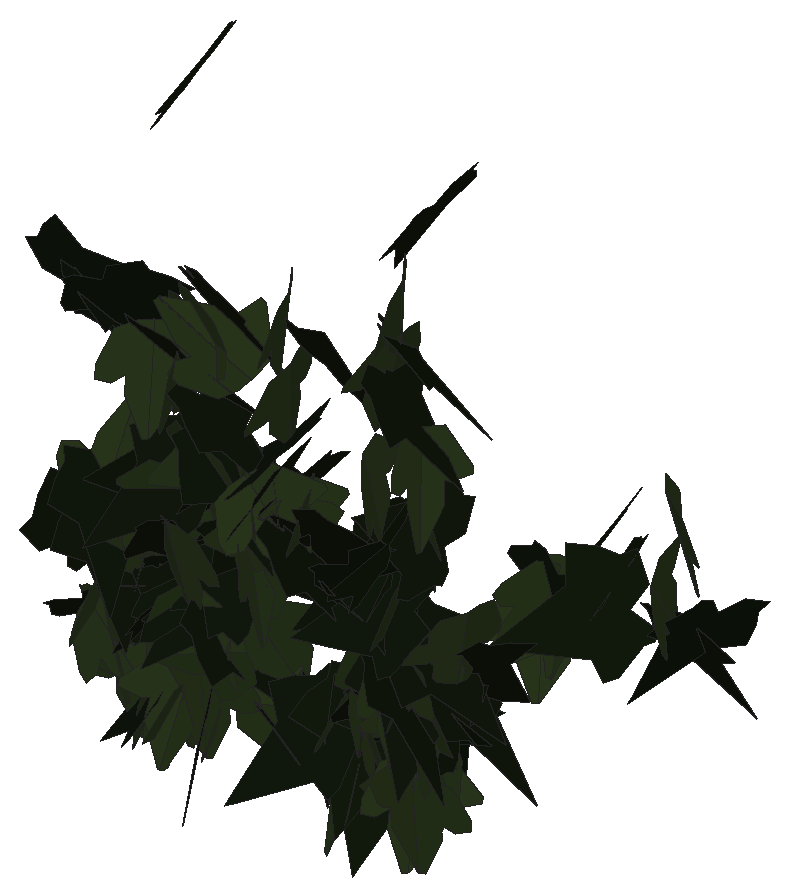
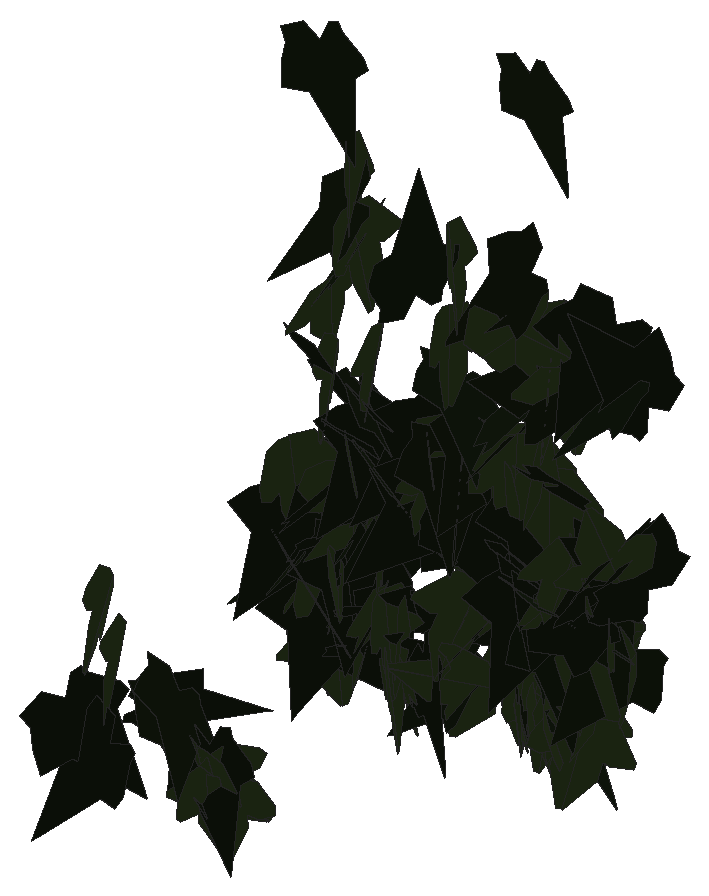
# SketchUp Ruby script. Lengths in inches.
U = 1.inch
M = Sketchup.active_model
def pt(a) = Geom::Point3d.new(a.map { |v| v * U })
def face(e, loops, mat)
  f = e.add_face(loops[0].map { |a| pt(a) })
  loops[1..].each { |l| e.add_face(l.map { |a| pt(a) }).erase! }
  f.material = f.back_material = mat if mat
  f
end
# faces: each face lists its corners as indices into pts; further lists are holes
def faces(e, pts, list, mat = nil) = list.each { |f| face(e, (f[0].is_a?(Array) ? f : [f]).map { |l| l.map { |i| pts[i] } }, mat) }
# xy, xz, yz: faces in a plane at the given z, y or x. An outline is a flat list of corners, or four numbers for a rectangle; further outlines are holes
def ring(l) = l.size == 4 ? [[l[0], l[1]], [l[2], l[1]], [l[2], l[3]], [l[0], l[3]]] : l.each_slice(2).to_a
def flat(e, list, mat, &to3) = list.each { |f| face(e, (f[0].is_a?(Array) ? f : [f]).map { |l| ring(l).map { |u, v| to3.(u, v) } }, mat) }
def xy(e, z, list, mat = nil) = flat(e, list, mat) { |x, y| [x, y, z] }
def xz(e, y, list, mat = nil) = flat(e, list, mat) { |x, z| [x, y, z] }
def yz(e, x, list, mat = nil) = flat(e, list, mat) { |y, z| [x, y, z] }
def lines(e, pts, list) = list.each { |a, b| e.add_line(pt(pts[a]), pt(pts[b])) }
# prism: a flat outline (further loops are holes) pulled along v
def prism(e, loops, v, mat = nil)
  f = face(e, loops, mat); d = Geom::Vector3d.new(v.map { |x| x * U })
  f.pushpull(f.normal.samedirection?(d) ? d.length : -d.length)
end
def box(e, o, s, mat = nil) = prism(e, [[o, [o[0] + s[0], o[1], o[2]], [o[0] + s[0], o[1] + s[1], o[2]], [o[0], o[1] + s[1], o[2]]]], [0, 0, s[2]], mat)
def at(x, y, z, deg = 0) = Geom::Transformation.translation(pt([x, y, z])) * Geom::Transformation.rotation(ORIGIN, Z_AXIS, deg.degrees)
def axes(o, x, y, z) = Geom::Transformation.new([*x, 0, *y, 0, *z, 0, *pt(o).to_a, 1])
def part(name) = M.definitions.add(name)
# library, detail: a bought-in or finely detailed component or shape, given as its bounding box
def library(name, o, s) = part(name).tap { |d| box(d.entities, o, s) }
def detail(e, o, s) = box(e.add_group.entities, o, s)
def put(e, d, t, mat = nil) = e.add_instance(d, t).tap { |i| i.material = mat if mat }
def group(e, t, mat = nil) = e.add_group.tap { |g| g.transformation = t; g.material = mat if mat }.entities
root = M.entities
M.materials.add("efeu1").color = [18, 25, 13]
M.materials.add("efeu2").color = [43, 57, 29]
c1 = part("ivyleaf_9")
p = [[1.54,2.16,1.25],[1.36,2.04,1.19],[-0.21,0.99,0.68],[-0.71,1.11,0.82],[-0.85,0.86,0.67],[-0.8,0.17,0.21],
  [-0.9,-0.01,0.1],[-0.67,-0.16,-0.02],[-0.08,-0.08,-0.05],[-0.03,-0.6,-0.4],[0.65,-0.88,-0.66],[0.83,-0.6,-0.49],
  [1.29,-0.42,-0.43],[1.8125,-0.07,-0.26],[1.21,0.44,0.15]]
faces(c1.entities,p,[[0,1,2,3,4,5,6,7,8,9,10,11,12,13,14]],"efeu1")
c2 = part("ivyleaf_10")
p = [[0,0.5,-0.03],[-0.0625,2.02,-0.43],[-0.19,2.01,-0.46],[-0.54,1.05,-0.29],[-0.52,0.625,-0.18],[-0.83,0.76,-0.28],
  [-1.16,0.64,-0.33],[-1.15,0.33,-0.24],[-0.77,-0.39,0.02],[-0.3,-0.51,0.16],[0.04,-0.48,0.23],[-0.02,2.01,-0.4375],
  [-0.06,2.01,-0.43],[0.04,-0.49,0.23],[0.67,-0.49,0.14],[1.38,0.36,-0.2],[1.375,0.51,-0.24],[0.81,0.65,-0.19],
  [0.62,0.59,-0.15],[0.6,1.09,-0.28],[0.5,1.23,-0.31]]
faces(c2.entities,p,[[0,1,2,3,4,5,6,7,8,9,10],[11,12,0,13,14,15,16,17,18,19,20]],"efeu2")
put(root,c1,axes([39.49,223.15,238.32],[0.47142,-0.1547,-0.06193],[0.05952,-0.01727,0.49614],[-0.15564,-0.47515,0.00213]))
put(root,c2,axes([37.74,222.87,235.76],[-0.47118,0.16717,0.00668],[-0.00578,0.00368,-0.49995],[-0.1672,-0.47121,-0.00153]))
put(root,c1,axes([38.08,222.8,241.44],[-0.21441,0.45128,0.01919],[-0.00987,0.01656,-0.49963],[-0.45158,-0.21463,0.00181]))
put(root,c1,axes([38.09,222.86,238.875],[0.48575,-0.11853,-0.00068],[0.00103,0.00709,-0.49995],[0.11853,0.4857,0.00713]))
put(root,c2,axes([36.67,222.96,234.79],[0.15334,-0.46907,-0.08039],[0.02982,0.09377,-0.49022],[0.47497,0.14555,0.05673]))
put(root,c2,axes([39.1,222.94,238.95],[0.18434,-0.44913,-0.11958],[-0.0031,0.12745,-0.48347],[0.46477,0.17899,0.04421]))
put(root,c2,axes([40.86,223.03,237.81],[0.04496,0.47796,-0.13977],[0.00326,-0.14061,-0.47981],[-0.49796,0.04223,-0.01576]))
put(root,c2,axes([38.29,223.1,237.94],[0.24274,0.2634,0.34886],[-0.24092,-0.25234,0.35816],[0.36474,-0.34197,0.00441]))
put(root,c1,axes([36.53,223.22,235.86],[0.05742,-0.49381,0.05339],[0.00046,-0.0537,-0.49711],[0.49669,0.05714,-0.00571]))
put(root,c1,axes([39.55,223.14,234.1],[-0.49666,-0.00558,0.05746],[-0.05747,0.00133,-0.49668],[0.00539,-0.49997,-0.00196]))
put(root,c2,axes([38.29,223.0625,234.56],[-0.15582,-0.01273,0.47493],[-0.45249,-0.14838,-0.15244],[0.14482,-0.47731,0.03473]))
put(root,c1,axes([41.11,222.88,240.86],[-0.15403,0.47011,-0.07259],[0.0126,-0.07224,-0.49459],[-0.47552,-0.1542,0.0104]))
put(root,c1,axes([36.91,222.76,238.54],[0.37466,0.32957,-0.0318],[-0.01735,-0.02842,-0.49889],[-0.33065,0.37493,-0.00986]))
put(root,c1,axes([39.125,222.98,236.22],[0.35353,-0.33498,-0.11316],[-0.03131,0.12973,-0.48186],[0.35218,0.34779,0.07075]))
put(root,c1,axes([37.91,223.23,233.9375],[-0.2139,0.074,-0.44584],[0.40905,-0.17803,-0.22579],[-0.19217,-0.46133,0.01563]))
put(root,c1,axes([40.63,223.08,235.85],[-0.43432,0.13698,0.2064],[-0.20798,0.02468,-0.45402],[-0.13457,-0.48024,0.03554]))
put(root,c1,axes([40.42,222.96,236.58],[-0.35188,0.35519,0.00467],[-0.00409,0.00251,-0.49998],[-0.35519,-0.3519,0.00114]))
put(root,c1,axes([37.67,223.2,236.49],[-0.49896,0.00205,0.03218],[-0.03223,-0.0447,-0.49695],[0.00084,-0.49799,0.04474]))
put(root,c2,axes([40.58,222.96,239.6],[0.17541,-0.43678,-0.16869],[-0.00356,0.17889,-0.46689],[0.46821,0.165,0.05965]))
put(root,c1,axes([40.46,222.96,238.57],[0.34199,-0.301,-0.20602],[-0.12245,0.17127,-0.45351],[0.34358,0.36065,0.04343]))
put(root,c2,axes([36.8,222.82,234.54],[0.04539,0.43983,0.23342],[0.00594,0.2339,-0.44188],[-0.4979,0.04289,0.01601]))
put(root,c2,axes([37.6,223.24,233.95],[-0.26932,-0.37968,0.18251],[0.0478,-0.24277,-0.43449],[0.41855,-0.21659,0.16706]))
put(root,c2,axes([37.29,223.04,237.82],[0.39107,0.31149,-0.00636],[-0.02897,0.02619,-0.49847],[-0.3102,0.39024,0.03853]))
put(root,c2,axes([40.4,223.12,238.8],[-0.00156,-0.49967,0.01823],[-0.00677,-0.0182,-0.49962],[0.49995,-0.00181,-0.00671]))
put(root,c1,axes([38.07,223.11,236.87],[0.20602,-0.43524,-0.13461],[-0.01776,0.13995,-0.47969],[0.45524,0.20243,0.04221]))
put(root,c2,axes([36.49,223.1,234.42],[-0.33295,0.28542,-0.24016],[0.19158,-0.14537,-0.43837],[-0.32007,-0.38393,-0.01256]))
put(root,c2,axes([39.87,223.26,234.97],[0.14736,-0.42313,0.22191],[0.22096,-0.14554,-0.42425],[0.42363,0.22311,0.1441]))
put(root,c2,axes([37.64,223.07,236.29],[-0.45741,-0.19272,0.06026],[-0.05386,-0.02735,-0.49634],[0.19461,-0.46055,0.00426]))
put(root,c1,axes([36.39,222.82,235.35],[-0.0583,-0.05927,0.49304],[0.41081,0.27314,0.08141],[-0.27899,0.41459,0.01685]))
put(root,c2,axes([38.74,222.95,236.56],[0.31773,0.28078,0.26497],[0.17044,0.20589,-0.42256],[-0.34641,0.35884,0.03512]))
put(root,c2,axes([40.39,223.16,235.91],[0.2238,-0.44659,-0.0217],[-0.00194,0.0233,-0.49945],[0.44711,0.22364,0.0087]))
put(root,c1,axes([37.3125,223.14,237.74],[0.34534,-0.22426,0.28363],[0.27768,-0.08672,-0.40666],[0.23159,0.43839,0.06465]))
put(root,c2,axes([38.58,223.09,235.83],[-0.11092,0.48323,-0.0647],[0.00446,-0.06534,-0.49569],[-0.48752,-0.11054,0.01019]))
put(root,c2,axes([38.08,222.96,238.18],[-0.03075,0.07711,-0.49306],[-0.42285,0.25833,0.06678],[0.26505,0.42109,0.04933]))
put(root,c1,axes([36.6,223.3,235.5],[0.00605,-0.49479,-0.07171],[-0.0052,0.07165,-0.49481],[0.49994,0.00673,-0.00428]))
put(root,c1,axes([36.07,223.22,238.0625],[0.05217,-0.08618,0.48975],[0.40505,-0.2783,-0.09212],[0.28847,0.40635,0.04078]))
put(root,c1,axes([37.92,223.11,237.35],[0.34648,-0.35591,-0.05723],[0.04335,0.11994,-0.48346],[0.35787,0.33006,0.11397]))
put(root,c1,axes([40.3,223.28,234.86],[0.23657,-0.43527,0.06766],[0.04729,-0.05126,-0.49511],[0.43795,0.24066,0.01691]))
put(root,c1,axes([38.2,223.28,235.34],[-0.49945,0.00762,-0.02217],[0.02189,-0.01738,-0.49922],[-0.00838,-0.49964,0.01702]))
put(root,c2,axes([37.64,222.97,237.76],[0.18603,-0.37182,-0.27775],[-0.02737,0.28992,-0.40644],[0.4633,0.16643,0.08752]))
put(root,c1,axes([40.52,223.02,239.02],[0.46272,-0.17673,-0.06824],[-0.03946,0.08623,-0.49093],[0.18529,0.45971,0.06585]))
put(root,c2,axes([37.9,223.03,236.74],[-0.47245,0.13857,0.0871],[-0.07933,0.03888,-0.49213],[-0.14317,-0.47884,-0.01475]))
put(root,c2,axes([40.2,223.01,237.33],[-0.18428,0.4437,0.13846],[-0.11988,0.09854,-0.47531],[-0.44908,-0.20838,0.07006]))
put(root,c2,axes([40.58,223.18,235.4],[-0.45472,-0.18508,0.09474],[-0.07997,-0.05462,-0.49053],[0.19193,-0.46126,0.02007]))
put(root,c2,axes([38.99,223.12,237.98],[0.03101,-0.47965,-0.13773],[0.01574,0.13887,-0.48007],[0.49879,0.02544,0.02371]))
put(root,c2,axes([40.68,223.15,233.68],[-0.48835,-0.09831,0.04298],[-0.03676,-0.03487,-0.49743],[0.1008,-0.489,0.02683]))
put(root,c2,axes([37.97,223.21,236.68],[-0.30479,-0.39612,-0.01404],[0.06394,-0.03165,-0.49488],[0.39117,-0.30346,0.06995]))
put(root,c1,axes([41.06,223.06,236.79],[-0.29122,0.24946,0.32087],[-0.26032,0.18866,-0.38294],[-0.31213,-0.3901,0.01999]))
put(root,c2,axes([40.42,223.14,235.11],[-0.46389,0.12989,0.13394],[-0.14721,-0.03428,-0.47661],[-0.11463,-0.48162,0.07005]))
put(root,c1,axes([37.7,222.92,235.96],[0.18086,0.46614,-0.00225],[0.00124,-0.00289,-0.49999],[-0.46614,0.18085,-0.0022]))
put(root,c2,axes([38.27,223.2,236.42],[0.42392,-0.2643,0.02104],[0.0862,0.09987,-0.48228],[0.25073,0.41252,0.13024]))
put(root,c1,axes([39.02,222.93,237.17],[-0.0745,0.46996,0.15359],[-0.11048,0.13558,-0.46842],[-0.48192,-0.10373,0.08364]))
put(root,c2,axes([37.85,223.2,234.03],[-0.46678,-0.1768,0.0292],[-0.01645,-0.03886,-0.49822],[0.17844,-0.46608,0.03046]))
put(root,c2,axes([37.02,223.29,235.6],[0.33719,-0.36899,0.01228],[0.0284,0.00935,-0.49911],[0.3681,0.33728,0.02727]))
put(root,c1,axes([39.28,223.03,236.37],[0.49082,0.09389,0.01679],[0.01787,-0.00404,-0.49966],[-0.09369,0.49109,-0.00732]))
put(root,c2,axes([38.64,223.21,235.92],[-0.47175,-0.16456,0.01932],[-0.01579,-0.01339,-0.49957],[0.16494,-0.47195,0.00744]))
put(root,c1,axes([37.66,223.24,235],[-0.35666,0.31001,0.16335],[-0.23313,-0.03591,-0.44086],[-0.26162,-0.39064,0.17016]))
put(root,c2,axes([39.63,223.33,233.52],[0.35905,-0.34797,-0.00209],[-0.00183,0.00111,-0.5],[0.34797,0.35905,-0.00048]))
put(root,c1,axes([36.27,223.15,238.23],[0.43884,-0.21544,-0.10491],[-0.05863,0.11571,-0.48288],[0.23235,0.43611,0.07629]))
put(root,c1,axes([37.3,223.19,233.78],[-0.31103,0.39135,-0.0103],[0.00597,-0.00841,-0.49989],[-0.39144,-0.31109,0.00056]))
put(root,c1,axes([39.96,223,236.17],[0.38146,0.31932,0.05021],[0.04324,0.02656,-0.49742],[-0.32034,0.38383,-0.00736]))
put(root,c2,axes([37.48,223.33,233.67],[0.09691,-0.48891,-0.03964],[-0.02416,0.0356,-0.49815],[0.48992,0.09847,-0.01673]))
put(root,c2,axes([38.875,223.14,236.1875],[-0.32299,-0.16859,-0.34243],[0.30285,0.15981,-0.36434],[0.23229,-0.44276,-0.00112]))
put(root,c2,axes([40.3,223.3125,234.89],[0.15083,0.47191,-0.06749],[-0.02031,-0.06436,-0.49542],[-0.47628,0.15219,-0.00025]))
put(root,c1,axes([37.34,223.18,234.43],[-0.30018,0.05649,0.39586],[0.38968,-0.0697,0.30544],[0.08969,0.49188,-0.00218]))
put(root,c1,axes([40.42,223.5625,234.93],[-0.13816,-0.4805,-0.00513],[0.00453,0.00404,-0.49996],[0.48051,-0.1382,0.00324]))
put(root,c1,axes([38,223.21,234.85],[0.31287,-0.3131,-0.23255],[-0.07755,0.24222,-0.43048],[0.38223,0.30544,0.103]))
put(root,c2,axes([36.96,223.09,235.45],[-0.21685,-0.20429,-0.40155],[0.29279,0.27481,-0.29792],[0.34242,-0.36435,0.00044]))
put(root,c2,axes([39.05,223.37,236.42],[0.23859,-0.43903,-0.01799],[0.03918,0.04165,-0.49672],[0.43765,0.23562,0.05428]))
put(root,c2,axes([40.6875,223.23,237.01],[-0.35526,0.34346,0.07632],[-0.08573,0.02069,-0.49216],[-0.34124,-0.36277,0.04419]))
put(root,c1,axes([39.78,223.6,234.22],[-0.2531,-0.43005,-0.03151],[0.02995,0.01892,-0.49874],[0.43016,-0.25436,0.01619]))
put(root,c1,axes([38.55,223.39,235.81],[0.14542,0.21863,-0.4255],[-0.24111,-0.35061,-0.26255],[-0.41318,0.28155,0.00346]))
put(root,c1,axes([39.375,223.26,235.49],[0.49285,-0.08419,-0.00374],[-0.00384,-0.00029,-0.49999],[0.08419,0.49286,-0.00093]))
put(root,c1,axes([36.46,223.02,234.56],[0.36853,0.32231,0.10148],[-0.00475,0.15509,-0.47532],[-0.33788,0.34937,0.11737]))
put(root,c1,axes([38.62,223.34,233.71],[0.45144,-0.2146,-0.01209],[-0.0128,0.00124,-0.49983],[0.21456,0.4516,-0.00438]))
put(root,c2,axes([41.08,223.41,235.66],[-0.1234,-0.4844,-0.01125],[-0.00269,0.0123,-0.49984],[0.48453,-0.1233,-0.00564]))
put(root,c1,axes([39.97,223.4,236.01],[-0.43766,0.24108,0.01824],[-0.01543,0.0098,-0.49967],[-0.24128,-0.43793,-0.00114]))
put(root,c2,axes([37.04,223.61,233.82],[0.14683,-0.42927,0.21016],[0.05982,-0.20162,-0.45362],[0.4742,0.15835,-0.00785]))
put(root,c2,axes([36.92,223.4,233.84],[-0.47427,-0.1498,0.05128],[-0.03728,-0.05175,-0.49592],[0.15389,-0.47422,0.03792]))
put(root,c2,axes([37.65,223.27,234.92],[-0.2454,-0.37208,-0.22657],[0.12537,0.18873,-0.44572],[0.41721,-0.27556,0.00067]))
put(root,c1,axes([38.66,223.01,236.41],[0.04848,0.3867,0.31323],[0.04598,0.30988,-0.38969],[-0.49552,0.06659,-0.00551]))
put(root,c1,axes([40.55,223.36,235.43],[0.25482,-0.35935,-0.2365],[-0.01884,0.26529,-0.4234],[0.42978,0.22469,0.12166]))
put(root,c2,axes([36.48,223.26,235.74],[0.30242,0.34578,-0.19742],[0.13333,0.14566,0.45936],[0.37519,-0.33048,-0.00411]))
put(root,c1,axes([37.31,223.28,234.68],[-0.05457,0.49341,-0.05974],[0.0096,-0.05904,-0.49641],[-0.49692,-0.05533,-0.00303]))
put(root,c1,axes([38.85,223.17,236.26],[0.03762,0.11901,-0.48417],[-0.47601,0.15301,0.00062],[0.14832,0.46089,0.12482]))
put(root,c2,axes([40.28,223.6,234.58],[0.20713,-0.44639,0.08849],[0.05044,-0.0741,-0.4919],[0.45227,0.2127,0.01434]))
put(root,c2,axes([40.42,223.5625,234.48],[-0.17128,-0.46645,0.05559],[0.00621,-0.06141,-0.49618],[0.46971,-0.16928,0.02683]))
put(root,c2,axes([37.31,223.45,233.92],[-0.49015,0.09867,0.00441],[-0.01336,-0.0441,-0.49787],[-0.09786,-0.48818,0.04587]))
put(root,c1,axes([40.1,223.6,234.38],[0.20799,-0.15243,0.42837],[0.34159,-0.25852,-0.25785],[0.30009,0.39992,-0.0034]))
put(root,c2,axes([40.38,223.44,234.49],[-0.38583,-0.29255,-0.12471],[0.12063,0.04679,-0.48297],[0.29425,-0.40277,0.03447]))
put(root,c1,axes([36.77,223.29,235.1],[0.40818,0.06374,0.28165],[0.27884,0.03981,-0.41312],[-0.07509,0.49432,-0.00305]))
put(root,c2,axes([39.69,223.36,234.13],[-0.4111,0.19825,0.20418],[-0.18666,0.08295,-0.45637],[-0.21482,-0.45146,0.00581]))
put(root,c2,axes([40.38,223.51,233.61],[0.33236,0.3715,-0.03905],[-0.04775,-0.00959,-0.49762],[-0.37048,0.33451,0.02911]))
put(root,c1,axes([39.78,223.75,233.75],[-0.25893,-0.42189,-0.07045],[0.08096,0.03252,-0.49233],[0.42,-0.26636,0.05147]))
put(root,c2,axes([38.91,223.35,236.27],[0.01591,0.47837,0.14461],[-0.008,0.14491,-0.47847],[-0.49968,0.01291,0.01226]))
put(root,c2,axes([37.03,223.38,235.81],[0.07472,0.4805,0.11633],[-0.00068,0.11775,-0.48594],[-0.49439,0.07246,0.01825]))
put(root,c1,axes([40.2,223.29,234.68],[0.16281,0.46937,-0.05638],[-0.05497,-0.04043,-0.49532],[-0.46954,0.16749,0.03844]))
put(root,c2,axes([40.67,223.43,234.23],[-0.10083,0.47853,0.10415],[-0.04239,0.0974,-0.48858],[-0.48789,-0.10735,0.02093]))
put(root,c2,axes([36.75,223.53,234.32],[-0.49821,0.04132,0.00917],[-0.0092,0.00003,-0.49992],[-0.04131,-0.49829,0.00073]))
put(root,c1,axes([38.98,223.3,235.8],[0.4245,0.2322,0.12603],[0.09848,0.08226,-0.48325],[-0.24516,0.43511,0.0241]))
put(root,c2,axes([39.55,223.57,234.25],[0.0579,-0.48625,-0.10104],[-0.01029,0.10053,-0.48968],[0.49653,0.05878,0.00163]))
put(root,c2,axes([39.84,223.45,234.1875],[-0.16426,0.44871,0.14724],[-0.06902,0.13141,-0.47746],[-0.46718,-0.17718,0.01877]))
put(root,c1,axes([38.82,223.375,236.47],[-0.02921,0.49739,0.04188],[0.00189,0.04206,-0.49822],[-0.49914,-0.02895,-0.00434]))
put(root,c2,axes([38.49,223.38,234.7],[0.2329,0.35528,0.26369],[-0.03253,0.31093,-0.39021],[-0.44125,0.16461,0.16795]))
put(root,c2,axes([37.83,223.375,233.68],[0.06126,-0.1294,-0.47906],[-0.23225,0.41909,-0.1429],[0.43853,0.24003,-0.00876]))
put(root,c2,axes([36.64,223.64,233.74],[-0.44533,-0.20627,-0.09556],[0.10393,0.0022,-0.48907],[0.20218,-0.45547,0.04092]))
put(root,c2,axes([40.45,223.55,234.375],[-0.41793,0.25174,0.10938],[-0.08799,0.06586,-0.48777],[-0.25999,-0.42695,-0.01075]))
put(root,c2,axes([39.42,223.68,233.62],[0.20145,-0.44921,-0.08735],[0.00519,0.09768,-0.49034],[0.45759,0.19665,0.04402]))
put(root,c1,axes([40.74,223.7,234.7],[0.32891,-0.37038,-0.0681],[0.02097,0.10829,-0.48768],[0.376,0.31795,0.08677]))
put(root,c2,axes([38.28,223.61,233.73],[0.0116,-0.02403,-0.49929],[0.49642,0.05913,0.00869],[0.05863,-0.49591,0.02523]))
put(root,c1,axes([37.39,223.46,235.15],[0.32685,0.37801,-0.01658],[-0.0084,-0.01466,-0.49971],[-0.37828,0.32695,-0.00324]))
put(root,c1,axes([39.05,223.55,233.77],[0.097,0.03103,-0.48952],[-0.49021,0.02331,-0.09566],[0.01688,0.49849,0.03494]))
put(root,c1,axes([40.87,223.57,234.29],[-0.246,0.30562,0.30996],[-0.17964,0.25303,-0.39205],[-0.3965,-0.30425,-0.01469]))
put(root,c1,axes([40.85,223.51,235.01],[0.2737,0.39812,0.12881],[0.07445,0.10513,-0.48312],[-0.41176,0.28364,-0.00173]))
put(root,c1,axes([40.29,223.65,234.16],[0.25883,0.42768,-0.00987],[-0.00479,-0.00864,-0.4999],[-0.42777,0.25887,-0.00038]))
put(root,c1,axes([40.44,226.84,234.14],[-0.33473,-0.15444,0.33779],[-0.29922,-0.15727,-0.36842],[0.22005,-0.44879,0.01286]))
put(root,c2,axes([41.09,226.63,234.63],[-0.15666,0.31123,0.3586],[-0.24793,0.26843,-0.34129],[-0.40496,-0.28474,0.07022]))
put(root,c2,axes([39.25,227.17,233.79],[0.2441,0.29768,-0.31907],[-0.23499,-0.21838,-0.38352],[-0.36769,0.33719,0.03329]))
put(root,c1,axes([40.2,226.95,234.3],[-0.26381,0.4245,0.01423],[-0.01219,0.00918,-0.49977],[-0.42457,-0.26403,0.00551]))
put(root,c2,axes([41.03,226.97,235.45],[-0.35548,0.34902,0.04263],[-0.03059,0.02969,-0.49818],[-0.35028,-0.35679,0.00025]))
put(root,c2,axes([39.37,227.18,233.92],[0.46791,-0.16729,0.05541],[0.05531,-0.00987,-0.49683],[0.16733,0.47108,0.00927]))
put(root,c2,axes([39.13,227.13,233.59],[0.44878,0.21934,0.02206],[0.01954,0.01027,-0.49951],[-0.21957,0.44921,0.00064]))
put(root,c1,axes([39.37,227.09,234.03],[0.26973,0.10108,-0.40869],[-0.37927,-0.15237,-0.28799],[-0.18277,0.46537,-0.00553]))
put(root,c1,axes([41.23,227.35,234.12],[-0.12626,0.32642,-0.35708],[-0.01165,-0.37099,-0.33501],[-0.48365,-0.07628,0.10129]))
put(root,c1,axes([39.89,227.02,234.54],[-0.07769,0.44917,0.20544],[-0.03426,0.20257,-0.45584],[-0.49274,-0.0849,-0.0007]))
put(root,c1,axes([40.62,227.42,233.79],[0.49484,0.01129,-0.07078],[-0.07068,-0.00506,-0.49495],[-0.0119,0.49985,-0.00341]))
